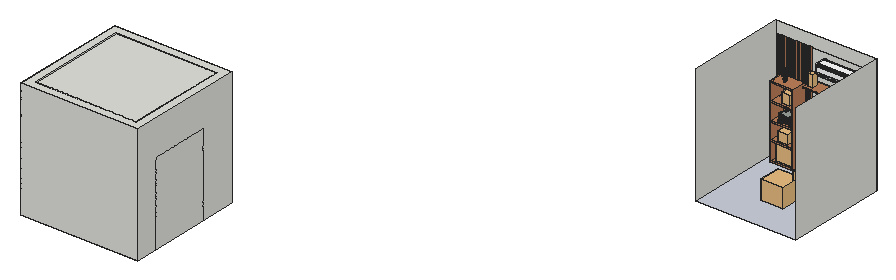
# SketchUp Ruby script. Lengths in inches.
U = 1.inch
M = Sketchup.active_model
def pt(a) = Geom::Point3d.new(a.map { |v| v * U })
def face(e, loops, mat)
  f = e.add_face(loops[0].map { |a| pt(a) })
  loops[1..].each { |l| e.add_face(l.map { |a| pt(a) }).erase! }
  f.material = f.back_material = mat if mat
  f
end
# faces: each face lists its corners as indices into pts; further lists are holes
def faces(e, pts, list, mat = nil) = list.each { |f| face(e, (f[0].is_a?(Array) ? f : [f]).map { |l| l.map { |i| pts[i] } }, mat) }
# xy, xz, yz: faces in a plane at the given z, y or x. An outline is a flat list of corners, or four numbers for a rectangle; further outlines are holes
def ring(l) = l.size == 4 ? [[l[0], l[1]], [l[2], l[1]], [l[2], l[3]], [l[0], l[3]]] : l.each_slice(2).to_a
def flat(e, list, mat, &to3) = list.each { |f| face(e, (f[0].is_a?(Array) ? f : [f]).map { |l| ring(l).map { |u, v| to3.(u, v) } }, mat) }
def xy(e, z, list, mat = nil) = flat(e, list, mat) { |x, y| [x, y, z] }
def xz(e, y, list, mat = nil) = flat(e, list, mat) { |x, z| [x, y, z] }
def yz(e, x, list, mat = nil) = flat(e, list, mat) { |y, z| [x, y, z] }
def lines(e, pts, list) = list.each { |a, b| e.add_line(pt(pts[a]), pt(pts[b])) }
# prism: a flat outline (further loops are holes) pulled along v
def prism(e, loops, v, mat = nil)
  f = face(e, loops, mat); d = Geom::Vector3d.new(v.map { |x| x * U })
  f.pushpull(f.normal.samedirection?(d) ? d.length : -d.length)
end
def box(e, o, s, mat = nil) = prism(e, [[o, [o[0] + s[0], o[1], o[2]], [o[0] + s[0], o[1] + s[1], o[2]], [o[0], o[1] + s[1], o[2]]]], [0, 0, s[2]], mat)
def at(x, y, z, deg = 0) = Geom::Transformation.translation(pt([x, y, z])) * Geom::Transformation.rotation(ORIGIN, Z_AXIS, deg.degrees)
def axes(o, x, y, z) = Geom::Transformation.new([*x, 0, *y, 0, *z, 0, *pt(o).to_a, 1])
def part(name) = M.definitions.add(name)
# library, detail: a bought-in or finely detailed component or shape, given as its bounding box
def library(name, o, s) = part(name).tap { |d| box(d.entities, o, s) }
def detail(e, o, s) = box(e.add_group.entities, o, s)
def put(e, d, t, mat = nil) = e.add_instance(d, t).tap { |i| i.material = mat if mat }
def group(e, t, mat = nil) = e.add_group.tap { |g| g.transformation = t; g.material = mat if mat }.entities
root = M.entities
M.materials.add("Book").color = [224, 222, 217]
M.materials.add("Color_000").color = [255, 255, 255]
M.materials.add("Gold_14k").color = [241, 247, 187]
M.materials.add("PDM_Books_04_Charcoal").color = [35, 35, 35]
M.materials.add("PDM_Books_04_Color_000").color = [255, 255, 255]
M.materials.add("PDM_Books_04_Color_D05").color = [255, 242, 204]
M.materials.add("PDM_Books_04_Material27").color = [78, 78, 71]
M.materials.add("PDM_Books_04_Material30").color = [128, 128, 127]
M.materials.add("PDM_Books_04_Material36").color = [212, 187, 166]
M.materials.add("PDM_Books_04_Material37").color = [155, 160, 155]
M.materials.add("PDM_Books_04_Material8").color = [90, 92, 88]
M.materials.add("[Color A05]").color = [234, 230, 226]
M.materials.add("[Color C02]").color = [238, 236, 225]
M.materials.add("[Color M06]").color = [86, 86, 86]
M.materials.add("[Color M09]").color = [0, 0, 0]
M.materials.add("[Color_A04]").color = [219, 164, 177]
M.materials.add("[Marble Carrara Floor Tile]").color = [204, 208, 219]
M.materials.add("[Wood Floor Dark]").color = [153, 94, 42]
M.materials.add("[Wood Veneer 02]").color = [190, 128, 91]
M.materials.add("bottom").color = [86, 95, 57]
c1 = library("download?mid=50c7180b9fccec56d493bfe20f94b6ab&ctyp=sp&cv=p8.",[149.43,43.83,17.86],[74.75,0.57,42.04])
c2 = library("Round+Table",[-6.7,-7.16,0],[19.69,19.69,24.5])
c3 = library("flowerpot",[-48.68,-51.05,0],[97.36,102.1,118.11])
c4 = part("Books_04_component_01")
xy(c4.entities,0,[[0.04,0,0,0.04,0,7.875,0.12,7.875,0.12,0.24,1.25,0.24,1.25,7.875,1.36,7.875,1.36,0.04,1.3125,0]],"PDM_Books_04_Color_000")
xy(c4.entities,0.11,[[0.12,0.24,0.12,7.76,0.21,7.74,0.3,7.73,0.4,7.73,0.49,7.72,0.87,7.72,0.96,7.73,1.06,7.73,1.15,7.74,1.25,7.76,1.25,0.24]],"PDM_Books_04_Color_D05")
xy(c4.entities,8.99,[[0.12,0.12,1.25,0.12,1.25,7.76,1.15,7.74,1.06,7.73,0.96,7.73,0.87,7.72,0.49,7.72,0.4,7.73,0.3,7.73,0.21,7.74,0.12,7.76]],"PDM_Books_04_Color_D05")
xy(c4.entities,9.1,[[0.04,0,1.3125,0,1.36,0.04,1.36,7.875,1.25,7.875,1.25,0.12,0.12,0.12,0.12,7.875,0,7.875,0,0.04]],"PDM_Books_04_Color_000")
xz(c4.entities,0,[[0.04,0,1.3125,9.1]],"PDM_Books_04_Material36")
xz(c4.entities,0.12,[[0.12,8.99,1.25,9.1]],"PDM_Books_04_Color_000")
xz(c4.entities,0.24,[[0.12,0,1.25,0.11]],"PDM_Books_04_Color_000")
xz(c4.entities,7.72,[[0.49,0.11,0.59,8.99],[0.59,0.11,0.68,8.99],[0.68,0.11,0.78,8.99],[0.78,0.11,0.87,8.99]],"PDM_Books_04_Color_D05")
xz(c4.entities,7.73,[[0.3,0.11,0.4,8.99],[0.96,0.11,1.06,8.99]],"PDM_Books_04_Color_D05")
xz(c4.entities,7.875,[[0,0,0.12,9.1],[1.25,0,1.36,9.1]],"PDM_Books_04_Color_000")
yz(c4.entities,0,[[0.04,0,7.875,9.1]],"PDM_Books_04_Material36")
yz(c4.entities,0.12,[[0.24,0,7.875,0,7.875,9.1,0.12,9.1,0.12,8.99,7.76,8.99,7.76,0.11,0.24,0.11]],"PDM_Books_04_Color_000")
yz(c4.entities,1.25,[[0.24,0,0.24,0.11,7.76,0.11,7.76,8.99,0.12,8.99,0.12,9.1,7.875,9.1,7.875,0]],"PDM_Books_04_Color_000")
yz(c4.entities,1.36,[[0.04,0,7.875,9.1]],"PDM_Books_04_Material36")
p = [[0.04,0,0],[0.04,0,9.1],[0,0.04,9.1],[0,0.04,0],[1.3125,0,9.1],[1.3125,0,0],
  [1.36,0.04,0],[1.36,0.04,9.1],[0.21,7.74,0.11],[0.12,7.76,0.11],[0.12,7.76,8.99],[0.21,7.74,8.99],
  [0.3,7.73,0.11],[0.3,7.73,8.99],[0.49,7.72,0.11],[0.4,7.73,0.11],[0.4,7.73,8.99],[0.49,7.72,8.99],
  [0.96,7.73,0.11],[0.87,7.72,0.11],[0.87,7.72,8.99],[0.96,7.73,8.99],[1.15,7.74,0.11],[1.06,7.73,0.11],
  [1.06,7.73,8.99],[1.15,7.74,8.99],[1.25,7.76,0.11],[1.25,7.76,8.99]]
faces(c4.entities,p,[[0,1,2,3],[4,5,6,7]],"PDM_Books_04_Material36")
faces(c4.entities,p,[[8,9,10,11],[12,8,11,13],[14,15,16,17],[18,19,20,21],[22,23,24,25],[26,22,25,27]],"PDM_Books_04_Color_D05")
c5 = part("Books_04_component_05")
xy(c5.entities,0,[[0.04,0,0,0.04,0,8.31,0.12,8.31,0.12,0.24,0.83,0.18,0.83,8.31,0.94,8.31,0.94,0.04,0.9,0]],"PDM_Books_04_Color_000")
xy(c5.entities,0.11,[[0.83,0.18,0.12,0.24,0.12,8.1875,0.17,8.18,0.23,8.18,0.29,8.17,0.35,8.17,0.41,8.16,0.53,8.16,0.59,8.17,0.65,8.17,0.71,8.18,0.77,8.18,0.83,8.1875]],"PDM_Books_04_Color_D05")
xy(c5.entities,9.65,[[0.12,0.24,0.83,0.24,0.83,8.1875,0.77,8.18,0.71,8.18,0.65,8.17,0.59,8.17,0.53,8.16,0.41,8.16,0.35,8.17,0.29,8.17,0.23,8.18,0.17,8.18,0.12,8.1875]],"PDM_Books_04_Color_D05")
xy(c5.entities,9.76,[[0.04,0,0.9,0,0.94,0.04,0.94,8.31,0.83,8.31,0.83,0.24,0.12,0.24,0.12,8.31,0,8.31,0,0.04]],"PDM_Books_04_Color_000")
xz(c5.entities,0,[[0.04,0,0.9,9.76]],"PDM_Books_04_Material37")
xz(c5.entities,0.24,[[0.12,9.65,0.83,9.76]],"PDM_Books_04_Color_000")
xz(c5.entities,8.16,[[0.41,0.11,0.47,9.65],[0.47,0.11,0.53,9.65]],"PDM_Books_04_Color_D05")
xz(c5.entities,8.17,[[0.29,0.11,0.35,9.65],[0.59,0.11,0.65,9.65]],"PDM_Books_04_Color_D05")
xz(c5.entities,8.18,[[0.17,0.11,0.23,9.65],[0.71,0.11,0.77,9.65]],"PDM_Books_04_Color_D05")
xz(c5.entities,8.31,[[0,0,0.12,9.76],[0.83,0,0.94,9.76]],"PDM_Books_04_Color_000")
yz(c5.entities,0,[[0.04,0,8.31,9.76]],"PDM_Books_04_Material37")
yz(c5.entities,0.12,[[0.24,0,8.31,0,8.31,9.76,0.24,9.76,0.24,9.65,8.1875,9.65,8.1875,0.11,0.24,0.11]],"PDM_Books_04_Color_000")
yz(c5.entities,0.83,[[0.18,0,0.18,0.11,8.1875,0.11,8.1875,9.65,0.24,9.65,0.24,9.76,8.31,9.76,8.31,0]],"PDM_Books_04_Color_000")
yz(c5.entities,0.94,[[0.04,0,8.31,9.76]],"PDM_Books_04_Material37")
p = [[0,0.04,9.76],[0,0.04,0],[0.04,0,0],[0.04,0,9.76],[0.94,0.04,0],[0.94,0.04,9.76],
  [0.9,0,9.76],[0.9,0,0],[0.83,0.18,0.11],[0.83,0.18,0],[0.12,0.24,0],[0.12,0.24,0.11],
  [0.12,8.1875,0.11],[0.12,8.1875,9.65],[0.17,8.18,9.65],[0.17,8.18,0.11],[0.29,8.17,0.11],[0.23,8.18,0.11],
  [0.23,8.18,9.65],[0.29,8.17,9.65],[0.41,8.16,0.11],[0.35,8.17,0.11],[0.35,8.17,9.65],[0.41,8.16,9.65],
  [0.59,8.17,0.11],[0.53,8.16,0.11],[0.53,8.16,9.65],[0.59,8.17,9.65],[0.71,8.18,0.11],[0.65,8.17,0.11],
  [0.65,8.17,9.65],[0.71,8.18,9.65],[0.83,8.1875,0.11],[0.77,8.18,0.11],[0.77,8.18,9.65],[0.83,8.1875,9.65]]
faces(c5.entities,p,[[0,1,2,3],[4,5,6,7]],"PDM_Books_04_Material37")
faces(c5.entities,p,[[8,9,10,11]],"PDM_Books_04_Color_000")
faces(c5.entities,p,[[12,13,14,15],[16,17,18,19],[20,21,22,23],[24,25,26,27],[28,29,30,31],[32,33,34,35]],"PDM_Books_04_Color_D05")
c6 = part("Books_04_component_02")
xy(c6.entities,0,[[0.04,0,0,0.04,0,7.67,0.12,7.67,0.12,0.12,1.11,0.12,1.11,7.67,1.22,7.67,1.22,0.04,1.18,0]],"PDM_Books_04_Color_000")
xy(c6.entities,0.08,[[0.12,0.12,1.11,7.59]],"PDM_Books_04_Color_D05")
xy(c6.entities,10.875,[[0.12,0.12,1.11,7.59]],"PDM_Books_04_Color_D05")
xy(c6.entities,10.99,[[0.04,0,1.18,0,1.22,0.04,1.22,7.67,1.11,7.67,1.11,0.12,0.12,0.12,0.12,7.67,0,7.67,0,0.04]],"PDM_Books_04_Color_000")
xz(c6.entities,0,[[0.04,0,1.18,10.99]],"PDM_Books_04_Material8")
xz(c6.entities,0.12,[[0.12,0,1.11,0.08],[0.12,0.08,1.11,10.875]])
xz(c6.entities,0.12,[[0.12,10.875,1.11,10.99]],"PDM_Books_04_Color_000")
xz(c6.entities,7.59,[[0.12,0.08,1.11,10.875]],"PDM_Books_04_Color_D05")
xz(c6.entities,7.67,[[1.11,0,1.22,10.99]],"PDM_Books_04_Color_000")
xz(c6.entities,7.67,[[0,0,0.12,10.99]],"PDM_Books_04_Material8")
yz(c6.entities,0,[[0.04,0,7.67,10.99]],"PDM_Books_04_Material8")
yz(c6.entities,0.12,[[0.12,0,7.67,0,7.67,10.99,0.12,10.99,0.12,10.875,7.59,10.875,7.59,0.08,0.12,0.08]])
yz(c6.entities,0.12,[[0.12,0.08,7.59,10.875]],"PDM_Books_04_Material8")
yz(c6.entities,1.11,[[0.12,0,0.12,0.08,7.59,0.08,7.59,10.875,0.12,10.875,0.12,10.99,7.67,10.99,7.67,0],[0.12,0.08,7.59,10.875]])
yz(c6.entities,1.22,[[0.04,0,7.67,10.99]],"PDM_Books_04_Material8")
p = [[0,0.04,10.99],[0,0.04,0],[0.04,0,0],[0.04,0,10.99],[1.22,0.04,0],[1.22,0.04,10.99],
  [1.18,0,10.99],[1.18,0,0]]
faces(c6.entities,p,[[0,1,2,3],[4,5,6,7]],"PDM_Books_04_Material8")
c7 = part("Books_04_component_03")
xy(c7.entities,0,[[0.04,0,0,0.04,0,7.67,0.12,7.67,0.12,0.12,1.11,0.12,1.11,7.67,1.22,7.67,1.22,0.04,1.18,0]],"PDM_Books_04_Color_000")
xy(c7.entities,0.08,[[0.12,0.12,1.11,7.59]],"PDM_Books_04_Color_D05")
xy(c7.entities,9.89,[[0.12,0.12,1.11,7.59]],"PDM_Books_04_Color_D05")
xy(c7.entities,10,[[0.04,0,1.18,0,1.22,0.04,1.22,7.67,1.11,7.67,1.11,0.12,0.12,0.12,0.12,7.67,0,7.67,0,0.04]],"PDM_Books_04_Color_000")
xz(c7.entities,0,[[0.04,7.99,1.18,10]],"PDM_Books_04_Color_000")
xz(c7.entities,0,[[0.04,0,1.18,7.99]],"PDM_Books_04_Material30")
xz(c7.entities,0.12,[[0.12,0,1.11,0.08],[0.12,0.08,1.11,9.89]])
xz(c7.entities,0.12,[[0.12,9.89,1.11,10]],"PDM_Books_04_Color_000")
xz(c7.entities,7.59,[[0.12,0.08,1.11,9.89]],"PDM_Books_04_Color_D05")
xz(c7.entities,7.67,[[1.11,0,1.22,10]],"PDM_Books_04_Color_000")
xz(c7.entities,7.67,[[0,0,0.12,10]],"PDM_Books_04_Material8")
yz(c7.entities,0,[[0.04,0,7.67,10]],"PDM_Books_04_Material30")
yz(c7.entities,0.12,[[0.12,0,7.67,0,7.67,10,0.12,10,0.12,9.89,7.59,9.89,7.59,0.08,0.12,0.08]])
yz(c7.entities,0.12,[[0.12,0.08,7.59,9.89]],"PDM_Books_04_Material8")
yz(c7.entities,1.11,[[0.12,0,0.12,0.08,7.59,0.08,7.59,9.89,0.12,9.89,0.12,10,7.67,10,7.67,0],[0.12,0.08,7.59,9.89]])
yz(c7.entities,1.22,[[0.04,0,7.67,10]],"PDM_Books_04_Material30")
p = [[0.04,0,0],[0.04,0,7.99],[0,0.04,7.99],[0,0.04,0],[1.18,0,7.99],[1.18,0,0],
  [1.22,0.04,0],[1.22,0.04,7.99],[0.04,0,10],[0,0.04,10],[1.18,0,10],[1.22,0.04,10]]
faces(c7.entities,p,[[0,1,2,3],[4,5,6,7]],"PDM_Books_04_Material30")
faces(c7.entities,p,[[1,8,9,2],[10,4,7,11]],"PDM_Books_04_Color_000")
c8 = part("Books_04_component_04")
xy(c8.entities,0,[[0.04,0,0,0.04,0,8.1,0.12,8.1,0.12,0.12,1.11,0.12,1.11,8.1,1.22,8.1,1.22,0.04,1.18,0]],"PDM_Books_04_Color_000")
xy(c8.entities,0.08,[[0.12,0.12,1.11,8.02]],"PDM_Books_04_Color_D05")
xy(c8.entities,11.98,[[0.12,0.12,1.11,8.02]],"PDM_Books_04_Color_D05")
xy(c8.entities,12.09,[[0.04,0,1.18,0,1.22,0.04,1.22,8.1,1.11,8.1,1.11,0.12,0.12,0.12,0.12,8.1,0,8.1,0,0.04]],"PDM_Books_04_Color_000")
xz(c8.entities,0,[[0.04,7.96,1.18,12.09]],"PDM_Books_04_Charcoal")
xz(c8.entities,0,[[0.04,0,1.18,7.96]],"PDM_Books_04_Material27")
xz(c8.entities,0.12,[[0.12,0,1.11,0.08],[0.12,0.08,1.11,11.98]])
xz(c8.entities,0.12,[[0.12,11.98,1.11,12.09]],"PDM_Books_04_Color_000")
xz(c8.entities,8.02,[[0.12,0.08,1.11,11.98]],"PDM_Books_04_Color_D05")
xz(c8.entities,8.1,[[1.11,0,1.22,12.09]],"PDM_Books_04_Color_000")
xz(c8.entities,8.1,[[0,0,0.12,12.09]],"PDM_Books_04_Material8")
yz(c8.entities,0,[[0.04,0,8.1,12.09]],"PDM_Books_04_Material27")
yz(c8.entities,0.12,[[0.12,0,8.1,0,8.1,12.09,0.12,12.09,0.12,11.98,8.02,11.98,8.02,0.08,0.12,0.08]])
yz(c8.entities,0.12,[[0.12,0.08,8.02,11.98]],"PDM_Books_04_Material8")
yz(c8.entities,1.11,[[0.12,0,0.12,0.08,8.02,0.08,8.02,11.98,0.12,11.98,0.12,12.09,8.1,12.09,8.1,0],[0.12,0.08,8.02,11.98]])
yz(c8.entities,1.22,[[0.04,0,8.1,12.09]],"PDM_Books_04_Material27")
p = [[0,0.04,7.96],[0,0.04,0],[0.04,0,0],[0.04,0,7.96],[1.18,0,7.96],[1.18,0,0],
  [1.22,0.04,0],[1.22,0.04,7.96],[0,0.04,12.09],[0.04,0,12.09],[1.18,0,12.09],[1.22,0.04,12.09]]
faces(c8.entities,p,[[0,1,2,3],[4,5,6,7]],"PDM_Books_04_Material27")
faces(c8.entities,p,[[8,0,3,9],[10,4,7,11]],"PDM_Books_04_Charcoal")
c9 = part("Book")
put(c9.entities,c4,axes([4.875,-4.73,3.67],[0,0,1],[0.10106,0.99488,0],[-0.99488,0.10106,0]))
put(c9.entities,c5,axes([4.5,-4.91,5.03],[0,0,1],[0.17365,0.98481,0],[-0.98481,0.17365,0]))
put(c9.entities,c6,axes([4.85,-4.7,1.22],[0,0,1],[0.108,0.99415,0],[-0.99415,0.108,0]))
put(c9.entities,c7,axes([5.47,-3.69,2.45],[0,0,1],[-0.04711,0.99889,0],[-0.99889,-0.04711,0]))
put(c9.entities,c8,axes([6.6,-3.07,0],[0,0,1],[-0.15643,0.98769,0],[-0.98769,-0.15643,0]))
c10 = library("Vase with Flower",[-2.59,-2.59,0],[5.18,5.18,11.38])
c11 = part("stem")
p = [[8.92,1.38,83.34],[12.34,1.73,96.125],[8.32,0.48,83.4375],[8.19,2.35,83.4375],[11.85,2.6,96.21],[6.99,0.55,83.63],
  [10.86,0.86,96.39],[11.85,0.86,96.21],[6.86,2.43,83.63],[10.86,2.6,96.39],[6.26,1.53,83.73],[10.36,1.73,96.48],
  [16.61,1.73,120.56],[16.3,1.18,120.63],[16.3,2.28,120.63],[15.69,1.18,120.77],[15.69,2.28,120.77],[15.375,1.73,120.84],
  [21.36,1.47,144.07],[21.11,1.47,144.13],[21.49,1.6875,144.05],[21.36,1.91,144.07],[21.11,1.91,144.13],[20.99,1.6875,144.16]]
faces(c11.entities,p,[[0,1,2],[3,4,0],[1,0,4],[5,2,6],[7,2,1],[7,6,2],[8,9,3],[4,3,9],
  [5,6,10],[8,10,9],[11,10,6],[11,9,10],[7,1,12,13],[1,4,14,12],[7,13,15,6],[4,9,16,14],
  [6,15,17,11],[17,16,9,11],[18,19,15,13],[12,20,18,13],[20,12,14,21],[21,14,16,22],[19,23,17,15],[16,17,23,22]],"bottom")
faces(c11.entities,p,[[18,20,21,22,23,19]])
c12 = part("leaf")
xy(c12.entities,0,[[1.27,0.625,0,1.89,0,3.7,1.27,5.43,3.34,6.6875,3.34,1.02]],"bottom")
p = [[3.34,6.6875,0],[5.69,5.05,-0.75],[6.53,3.7,-1.02],[6.53,1.64,-1.02],[4.9375,0.625,-0.51],[3.34,1.02,0],
  [3.34,0.4375,0],[3.34,0,0]]
faces(c12.entities,p,[[0,1,2,3,4,5]],"bottom")
lines(c12.entities,p,[[5,6],[6,7]])
c13 = part("petal\#1")
p = [[0.59,-0.98,-0.45],[0.74,-1.1,-0.29],[0.41,-0.67,-0.14],[0.42,-0.77,-0.38],[1.2,-1.19,-0.06],[0.54,-0.34,0.24],
  [1.12,0.01,0.5],[1.78,-0.84,0.21],[1.45,-0.41,0.36],[0,0.42,0],[0.09,0.28,0.2],[0.09,0.84,0.2],
  [0,0.7,0],[1.87,-0.35,0.24],[2.18,-0.15,0.17],[2.39,0.2,0.15],[2.22,0.41,0.23],[1.85,0.28,0.32],
  [1.6,0,0.36],[0.45,0,0.45],[0.45,1.12,0.45],[1.87,0.28,0.35],[1.87,0.84,0.35],[2.23,0.7,0.23],
  [1.51,0.33,0.48],[1.16,0.56,0.6],[1.16,0,0.6],[1.51,0.79,0.48],[1.16,1.12,0.6]]
faces(c13.entities,p,[[0,1,2,3],[1,4,5,2],[6,5,4,7,8],[9,10,11,12],[13,8,7,14],[14,15,16,17,18,8,13],[10,19,20,11],[21,16,22],
  [23,22,16],[6,8,18,17],[24,25,26,21],[22,27,25,24,21],[28,25,27,22],[28,20,19,26,25]],"[Color_A04]")
c14 = part("flower")
put(c14.entities,c13,axes([2.1,0,0.625],[-0.03304,0.72958,0.14199],[-0.77918,0,-0.18132],[-0.17781,-0.15676,0.76408]))
put(c14.entities,c13,axes([3.38,2.1,1.25],[-0.77918,0,-0.18132],[0,-0.8,0],[-0.18132,0,0.77918]))
put(c14.entities,c13,axes([0.01,1.2,0],[0.7057,0,0.37681],[0,0.8,0],[-0.37681,0,0.7057]))
put(c14.entities,c13,axes([1.16,3.49,0.73],[0,-0.8,0],[0.77918,0,0.18132],[-0.18132,0,0.77918]))
c15 = part("Plant_flower")
p = [[4.13,-5.21,48.5625],[2.97,-5.27,48.18],[2.1,-5.33,47.33],[1.6875,-5.39,46.18],[2.87,-8.33,51.63],[2.46,-7.41,51.49],
  [2,-6.68,50.88],[1.58,-6.29,49.94]]
lines(c15.entities,p,[[0,1],[1,2],[2,3],[4,5],[6,7],[5,6]])
put(c15.entities,c11,axes([-0.85,0.55,-1.29],[0.10275,-0.38349,0],[0.38349,0.10275,0],[0,0,0.39701]))
put(c15.entities,c12,axes([3.82,-6.52,48.84],[0.09945,0.40738,-0.08753],[0.52591,-0.18667,-0.27125],[-0.22953,-0.03449,-0.42129]))
put(c15.entities,c14,axes([6.9,-4.04,53.68],[-2.40969,0.82543,0.59906],[-0.96837,-2.33406,-0.67913],[0.32013,-0.84712,2.45494]))
put(c15.entities,c12,axes([1.64,-8.47,52.18],[0.38389,0.04123,-0.17257],[-0.11872,-0.44244,-0.27916],[-0.18424,0.2028,-0.32786]))
c16 = part("stem2")
p = [[11.85,0.86,96.21],[12.34,1.73,96.125],[16.61,1.73,120.56],[16.3,1.18,120.63],[11.85,2.6,96.21],[16.3,2.28,120.63],
  [15.69,1.18,120.77],[10.86,0.86,96.39],[10.86,2.6,96.39],[15.69,2.28,120.77],[15.375,1.73,120.84],[10.36,1.73,96.48],
  [21.36,1.47,144.07],[21.11,1.47,144.13],[21.49,1.6875,144.05],[21.36,1.91,144.07],[21.11,1.91,144.13],[20.99,1.6875,144.16]]
faces(c16.entities,p,[[0,1,2,3],[1,4,5,2],[0,3,6,7],[4,8,9,5],[7,6,10,11],[10,9,8,11],[12,13,6,3],[2,14,12,3],
  [14,2,5,15],[15,5,9,16],[13,17,10,6],[9,10,17,16]],"bottom")
faces(c16.entities,p,[[12,14,15,16,17,13]])
c17 = part("Plant_flower2")
p = [[2.87,-8.33,51.63],[2.46,-7.41,51.49],[2,-6.68,50.88],[1.58,-6.29,49.94]]
lines(c17.entities,p,[[0,1],[2,3],[1,2]])
put(c17.entities,c16,axes([-0.85,0.55,-1.29],[0.10275,-0.38349,0],[0.38349,0.10275,0],[0,0,0.39701]))
put(c17.entities,c14,axes([6.9,-4.04,53.68],[-2.40969,0.82543,0.59906],[-0.96837,-2.33406,-0.67913],[0.32013,-0.84712,2.45494]))
put(c17.entities,c12,axes([1.64,-8.47,52.18],[0.38389,0.04123,-0.17257],[-0.11872,-0.44244,-0.27916],[-0.18424,0.2028,-0.32786]))
c18 = part("Vase_Quarter\#3")
xy(c18.entities,0,[[0,0,0,0.8,0.21,0.8,0.59,0.59,0.8,0.21,0.8,0]])
xz(c18.entities,0.78,[[0,9.66,0.21,10.84]])
yz(c18.entities,0.78,[[0,9.66,0.21,10.84]])
p = [[0.8,0,0],[0.8,0.21,0],[1.35,0.42,2.81],[1.35,0,2.81],[0.59,0.59,0],[1.01,1.01,2.81],
  [0.21,0.8,0],[0.42,1.35,2.81],[0,0.8,0],[0,1.35,2.81],[1.51,0.46,4.94],[1.51,0,4.94],
  [1.125,1.125,4.94],[0.46,1.51,4.94],[0,1.51,4.94],[1.43,0.43,6.19],[1.43,0,6.19],[1.07,1.07,6.19],
  [0.43,1.43,6.19],[0,1.43,6.19],[1,0.27,8.5],[1,0,8.5],[0.73,0.73,8.5],[0.27,1,8.5],
  [0,1,8.5],[0.78,0.21,9.66],[0.78,0,9.66],[0.57,0.57,9.66],[0.21,0.78,9.66],[0,0.78,9.66],
  [0.57,0.57,10.84],[0.78,0.21,10.84],[0.21,0.78,10.84],[1,0.27,12],[1,0,12],[0.78,0,10.84],
  [0.73,0.73,12],[0.27,1,12],[0,0.78,10.84],[0,1,12]]
faces(c18.entities,p,[[0,1,2,3],[4,5,2,1],[5,4,6,7],[7,6,8,9],[2,10,11,3],[5,12,10,2],[12,5,7,13],[13,7,9,14],
  [10,15,16,11],[12,17,15,10],[12,13,18,17],[13,14,19,18],[15,20,21,16],[17,22,20,15],[17,18,23,22],[18,19,24,23],
  [25,26,21,20],[22,27,25,20],[23,28,27,22],[23,24,29,28],[27,30,31,25],[28,32,30,27],[33,34,35,31],[30,36,33,31],
  [32,37,36,30],[32,38,39,37]])
c19 = part("vase_thin\#1")
put(c19.entities,c18,at(0,0,0))
put(c19.entities,c18,at(0,0,0,90))
put(c19.entities,c18,at(0,0,0,180))
put(c19.entities,c18,at(0,0,0,-90))
c20 = part("Vase with flowers")
put(c20.entities,c15,axes([3.625,2.02,-8.35],[-0.06695,-0.33202,0.02963],[0.33329,-0.0672,0],[0.00586,0.02905,0.33871]))
put(c20.entities,c15,axes([1.32,2.29,-9.75],[-0.088,0.32841,0],[-0.32841,-0.088,0],[0,0,0.34]))
put(c20.entities,c17,axes([3.73,4.01,-12],[0.14851,-0.30585,0],[0.30585,0.14851,0],[0,0,0.34]))
put(c20.entities,c19,axes([2.72,2.71,0],[1,0,0],[0,1,0],[0,0,0.44]))
put(c20.entities,c15,axes([2.75,3.98,-10.5],[0.33881,-0.02845,0],[0.02845,0.33881,0],[0,0,0.34]))
c21 = library("007",[-7.44,-2.67,-4.4375],[12.18,12.03,12.77])
c22 = library("skpE36B",[-3.84,-2.73,0],[7.68,5.46,1.59])
c23 = library("skpA613",[-33.11,-37.89,-86.79],[66.22,75.78,173.58])
c24 = library("Row of books",[-2.76,0,0],[10.13,7.78,9.38])
c25 = part("Open-Book2")
g1 = group(c25.entities,at(-83.63,0.99,-0.02))
g2 = group(g1,at(0,0,0))
xy(g2,0.028,[[0,0,2.913,10.029],[12.526,0,16.143,10.029]],"[Color M06]")
xy(g2,0.271,[[0.25,0,2.855,10.029]],"[Color A05]")
xy(g2,0.528,[[12.444,0,15.85,10.029]],"[Color C02]")
xz(g2,0,[[8.098,0,8.236,0.143,8.389,0.271,8.554,0.383,8.729,0.477,8.914,0.553,9.105,0.609,9.301,0.645,9.5,0.66,9.639,0.657,9.699,0.655,9.896,0.63,10.09,0.584,10.278,0.519,11,0.313,11.754,0.123,12.526,0.028,16.143,0.028,15.85,0.528,12.444,0.528,11.844,0.602,11.126,0.783,10.855,0.929,10.57,1.046,10.275,1.133,9.972,1.187,9.665,1.209,9.357,1.199,9.0625,1.158,9.052,1.156,8.753,1.082,8.464,0.976,8.1875,0.84,7.927,0.676,7.685,0.485,7.594,0.824,7.484,1.058,7.3,1.302,7.07,1.503,6.804,1.653,6.636,1.672,6.467,1.678,6.298,1.672,6.13,1.652,5.963,1.62,5.8,1.574,5.641,1.517,5.487,1.447,5.338,1.365,5.197,1.272,5.063,1.169,4.937,1.055,4.775,0.963,4.611,0.875,4.451,0.795,4.444,0.792,4.284,0.706,3.933,0.574,3.93,0.573,3.928,0.572,3.592,0.445,3.414,0.403,3.399,0.398,3.219,0.351,3.038,0.308,2.855,0.271,0.25,0.271,0,0.028,2.913,0.028,3.661,0.204,3.665,0.205,3.669,0.207,4.383,0.477,4.388,0.478,4.392,0.481,5.066,0.841,5.072,0.845,5.698,1.292,5.784,1.355,5.876,1.409,5.973,1.454,6.074,1.488,6.178,1.512,6.243,1.521,6.253,1.525,6.262,1.523,6.284,1.526,6.391,1.528,6.497,1.52,6.602,1.501,6.705,1.471,6.804,1.432,6.819,1.423,6.867,1.398,6.898,1.382,6.987,1.323,7.07,1.255,7.145,1.179,7.212,1.096,7.245,1.045,7.27,1.007,7.299,0.951,7.319,0.912,7.358,0.8125,7.387,0.71,7.405,0.605,7.413,0.498,7.413,0.497,7.409,0.391,7.395,0.286,7.37,0.182]],"Book")
xz(g2,10.029,[[8.098,0,7.37,0.182,7.395,0.286,7.409,0.391,7.413,0.497,7.413,0.498,7.405,0.605,7.387,0.71,7.358,0.8125,7.319,0.912,7.299,0.951,7.27,1.007,7.245,1.045,7.212,1.096,7.145,1.179,7.07,1.255,6.987,1.323,6.898,1.382,6.867,1.398,6.819,1.423,6.804,1.432,6.705,1.471,6.602,1.501,6.497,1.52,6.391,1.528,6.284,1.526,6.262,1.523,6.253,1.525,6.243,1.521,6.178,1.512,6.074,1.488,5.973,1.454,5.876,1.409,5.784,1.355,5.698,1.292,5.072,0.845,5.066,0.841,4.392,0.481,4.388,0.478,4.383,0.477,3.669,0.207,3.665,0.205,3.661,0.204,2.913,0.028,0,0.028,0.25,0.271,2.855,0.271,3.038,0.308,3.219,0.351,3.399,0.398,3.414,0.403,3.592,0.445,3.928,0.572,3.93,0.573,3.933,0.574,4.284,0.706,4.444,0.792,4.451,0.795,4.611,0.875,4.775,0.963,4.937,1.055,5.063,1.169,5.197,1.272,5.338,1.365,5.487,1.447,5.641,1.517,5.8,1.574,5.963,1.62,6.13,1.652,6.298,1.672,6.467,1.678,6.636,1.672,6.804,1.653,7.07,1.503,7.3,1.302,7.484,1.058,7.594,0.824,7.685,0.485,7.927,0.676,8.1875,0.84,8.464,0.976,8.753,1.082,9.052,1.156,9.0625,1.158,9.357,1.199,9.665,1.209,9.972,1.187,10.275,1.133,10.57,1.046,10.855,0.929,11.126,0.783,11.844,0.602,12.444,0.528,15.85,0.528,16.143,0.028,12.526,0.028,11.754,0.123,11,0.313,10.278,0.519,10.09,0.584,9.896,0.63,9.699,0.655,9.639,0.657,9.5,0.66,9.301,0.645,9.105,0.609,8.914,0.553,8.729,0.477,8.554,0.383,8.389,0.271,8.236,0.143]],"Book")
yz(g2,7.413,[[0,0.497,10.029,0.498]],"[Color M06]")
p = [[0,0,0.028],[0.25,0,0.271],[0.25,10.029,0.271],[0,10.029,0.028],[3.661,0,0.204],[2.913,0,0.028],
  [2.913,10.029,0.028],[3.661,10.029,0.204],[8.098,0,0],[7.37,0,0.182],[7.37,10.029,0.182],[8.098,10.029,0],
  [8.236,0,0.143],[8.236,10.029,0.143],[12.526,0,0.028],[11.754,0,0.123],[11.754,10.029,0.123],[12.526,10.029,0.028],
  [15.85,0,0.528],[16.143,0,0.028],[16.143,10.029,0.028],[15.85,10.029,0.528],[8.389,0,0.271],[8.389,10.029,0.271],
  [11,0,0.313],[11,10.029,0.313],[3.665,0,0.205],[3.665,10.029,0.205],[3.669,0,0.207],[3.669,10.029,0.207],
  [4.383,0,0.477],[4.383,10.029,0.477],[7.395,0,0.286],[7.395,10.029,0.286],[2.855,0,0.271],[3.038,0,0.308],
  [3.038,10.029,0.308],[2.855,10.029,0.271],[3.219,0,0.351],[3.219,10.029,0.351],[7.409,0,0.391],[7.409,10.029,0.391],
  [8.554,0,0.383],[8.554,10.029,0.383],[10.278,0,0.519],[10.278,10.029,0.519],[3.399,0,0.398],[3.399,10.029,0.398],
  [3.414,0,0.403],[3.592,0,0.445],[3.592,10.029,0.445],[3.414,10.029,0.403],[3.928,0,0.572],[3.928,10.029,0.572],
  [7.413,0,0.497],[7.413,10.029,0.497],[8.729,0,0.477],[8.729,10.029,0.477],[4.388,0,0.478],[4.388,10.029,0.478],
  [4.392,0,0.481],[4.392,10.029,0.481],[5.066,0,0.841],[5.066,10.029,0.841],[7.413,0,0.498],[7.405,0,0.605],
  [7.405,10.029,0.605],[7.413,10.029,0.498],[7.594,0,0.824],[7.685,0,0.485],[7.685,10.029,0.485],[7.594,10.029,0.824],
  [7.927,0,0.676],[7.927,10.029,0.676],[8.914,0,0.553],[8.914,10.029,0.553],[10.09,0,0.584],[10.09,10.029,0.584],
  [11.844,0,0.602],[12.444,0,0.528],[12.444,10.029,0.528],[11.844,10.029,0.602],[3.933,0,0.574],[4.284,0,0.706],
  [4.284,10.029,0.706],[3.933,10.029,0.574],[3.93,0,0.573],[3.93,10.029,0.573],[7.387,0,0.71],[7.387,10.029,0.71],
  [9.105,0,0.609],[9.105,10.029,0.609],[9.301,0,0.645],[9.301,10.029,0.645],[9.5,0,0.66],[9.5,10.029,0.66],
  [9.896,0,0.63],[9.699,0,0.655],[9.699,10.029,0.655],[9.896,10.029,0.63],[11.126,0,0.783],[11.126,10.029,0.783],
  [4.444,0,0.792],[4.444,10.029,0.792],[7.358,0,0.8125],[7.358,10.029,0.8125],[8.1875,0,0.84],[8.1875,10.029,0.84],
  [9.639,0,0.657],[9.639,10.029,0.657],[4.451,0,0.795],[4.451,10.029,0.795],[4.611,0,0.875],[4.611,10.029,0.875],
  [5.069,0,0.843],[5.069,10.029,0.843],[5.072,0,0.845],[5.072,10.029,0.845],[5.698,0,1.292],[5.698,10.029,1.292],
  [7.319,0,0.912],[7.319,10.029,0.912],[7.484,0,1.058],[7.484,10.029,1.058],[8.464,0,0.976],[8.464,10.029,0.976],
  [10.855,0,0.929],[10.855,10.029,0.929],[4.775,0,0.963],[4.775,10.029,0.963],[7.299,0,0.951],[7.299,10.029,0.951],
  [10.57,0,1.046],[10.57,10.029,1.046],[4.937,0,1.055],[4.937,10.029,1.055],[7.245,0,1.045],[7.212,0,1.096],
  [7.212,10.029,1.096],[7.245,10.029,1.045],[7.27,0,1.007],[7.27,10.029,1.007],[8.753,0,1.082],[8.753,10.029,1.082],
  [10.275,0,1.133],[10.275,10.029,1.133],[5.063,0,1.169],[5.063,10.029,1.169],[7.145,0,1.179],[7.145,10.029,1.179],
  [7.3,0,1.302],[7.3,10.029,1.302],[9.052,0,1.156],[9.052,10.029,1.156],[9.972,0,1.187],[9.972,10.029,1.187],
  [5.197,0,1.272],[5.197,10.029,1.272],[7.07,0,1.255],[7.07,10.029,1.255],[9.0625,0,1.158],[9.357,0,1.199],
  [9.357,10.029,1.199],[9.0625,10.029,1.158],[9.665,0,1.209],[9.665,10.029,1.209],[5.338,0,1.365],[5.338,10.029,1.365],
  [5.784,0,1.355],[5.784,10.029,1.355],[6.987,0,1.323],[6.898,0,1.382],[6.898,10.029,1.382],[6.987,10.029,1.323],
  [7.07,0,1.503],[7.07,10.029,1.503],[5.487,0,1.447],[5.487,10.029,1.447],[5.641,0,1.517],[5.641,10.029,1.517],
  [5.876,0,1.409],[5.876,10.029,1.409],[5.973,0,1.454],[5.973,10.029,1.454],[6.804,0,1.432],[6.705,0,1.471],
  [6.705,10.029,1.471],[6.804,10.029,1.432],[6.819,0,1.423],[6.819,10.029,1.423],[6.867,0,1.398],[6.867,10.029,1.398],
  [5.8,0,1.574],[5.8,10.029,1.574],[6.074,0,1.488],[6.074,10.029,1.488],[6.178,0,1.512],[6.178,10.029,1.512],
  [6.243,0,1.521],[6.243,10.029,1.521],[6.253,0,1.525],[6.253,10.029,1.525],[6.262,0,1.523],[6.262,10.029,1.523],
  [6.284,0,1.526],[6.284,10.029,1.526],[6.391,0,1.528],[6.391,10.029,1.528],[6.497,0,1.52],[6.497,10.029,1.52],
  [6.602,0,1.501],[6.602,10.029,1.501],[6.804,0,1.653],[6.804,10.029,1.653],[5.963,0,1.62],[5.963,10.029,1.62],
  [6.13,0,1.652],[6.13,10.029,1.652],[6.298,0,1.672],[6.298,10.029,1.672],[6.467,0,1.678],[6.467,10.029,1.678],
  [6.636,0,1.672],[6.636,10.029,1.672]]
faces(g2,p,[[0,1,2,3],[18,19,20,21]],"Book")
faces(g2,p,[[4,5,6,7],[8,9,10,11],[12,8,11,13],[14,15,16,17],[22,12,13,23],[15,24,25,16],[26,4,7,27],[28,26,27,29],
  [30,28,29,31],[9,32,33,10],[32,40,41,33],[42,22,23,43],[24,44,45,25],[40,54,55,41],[56,42,43,57],[58,30,31,59],
  [60,58,59,61],[62,60,61,63],[64,65,66,67],[74,56,57,75],[44,76,77,45],[65,88,89,66],[90,74,75,91],[92,90,91,93],
  [94,92,93,95],[96,97,98,99],[76,96,99,77],[88,104,105,89],[108,94,95,109],[97,108,109,98],[114,62,63,115],[116,114,115,117],
  [118,116,117,119],[104,120,121,105],[120,130,131,121],[136,137,138,139],[140,136,139,141],[130,140,141,131],[137,148,149,138],[148,158,159,149],
  [168,118,119,169],[170,171,172,173],[158,170,173,159],[180,168,169,181],[182,180,181,183],[184,185,186,187],[188,184,187,189],[190,188,189,191],
  [171,190,191,172],[194,182,183,195],[196,194,195,197],[198,196,197,199],[200,198,199,201],[202,200,201,203],[204,202,203,205],[206,204,205,207],
  [208,206,207,209],[210,208,209,211],[185,210,211,186]],"[Color M06]")
faces(g2,p,[[34,35,36,37],[35,38,39,36],[38,46,47,39],[48,49,50,51],[46,48,51,47],[49,52,53,50],[68,69,70,71],[82,83,84,85],
  [86,82,85,87],[52,86,87,53],[83,102,103,84],[102,110,111,103],[110,112,113,111],[122,68,71,123],[112,128,129,113],[128,134,135,129],
  [134,146,147,135],[150,122,123,151],[146,156,157,147],[156,166,167,157],[174,150,151,175],[166,176,177,167],[176,178,179,177],[178,192,193,179],
  [212,174,175,213],[192,214,215,193],[214,216,217,215],[216,218,219,217],[218,220,221,219],[220,222,223,221],[222,212,213,223]],"[Color A05]")
faces(g2,p,[[69,72,73,70],[78,79,80,81],[100,78,81,101],[72,106,107,73],[106,124,125,107],[126,100,101,127],[132,126,127,133],[124,142,143,125],
  [144,132,133,145],[142,152,153,143],[154,144,145,155],[160,161,162,163],[152,160,163,153],[161,164,165,162],[164,154,155,165]],"[Color C02]")
c26 = part("Air-conditioning")
g3 = group(c26.entities,at(10.25,0,0,90))
xy(g3,0,[[0,0.37,46.46,0.41],[0,0.41,46.46,4.01]],"Color_000")
xy(g3,12.99,[[0,0.47,46.46,0.54]])
xy(g3,12.99,[[0,0.54,46.46,8.38]],"Color_000")
xz(g3,0,[[0,12.45,46.46,12.52]])
xz(g3,0,[[0,0.35,46.46,12.45]],"Color_000")
xz(g3,10.25,[[[0,5.71,46.46,11.16],[0.95,6.51,45.74,10.625]],[0.95,6.51,45.74,10.625]],"Color_000")
yz(g3,0,[[0.37,0,0.32,0.01,0.27,0.03,0.23,0.04,0.18,0.07,0.14,0.1,0.11,0.13,0.05,0.21,0.03,0.25,0.01,0.3,0,0.35,0,12.52,0.04,12.66,0.07,12.72,0.11,12.78,0.21,12.88,0.27,12.92,0.34,12.95,0.4,12.98,0.47,12.99,8.38,12.99,8.62,12.98,8.86,12.93,9.09,12.85,9.31,12.75,9.51,12.62,9.69,12.46,9.85,12.28,9.99,12.08,10.1,11.86,10.18,11.63,10.23,11.4,10.25,11.16,10.25,5.71,7.36,1.21,7.125,1.02,6.875,0.85,6.62,0.69,6.35,0.55,6.07,0.42,5.79,0.3125,5.5,0.22,5.21,0.14,4.91,0.08,4.61,0.03,4.31,0.01,4.01,0]],"Color_000")
yz(g3,1.69,[[8.12,2.39,8.43,2.87,8.09,3.39,7.65,2.69],[8.67,2.5,8.43,2.87,8.5,2.97,8.73,2.625],[8.43,2.87,8.5,2.97,8.16,3.49,8.09,3.39],[8.5,2.97,9.19,4.05,8.72,4.36,8.16,3.49],[8.09,3.39,7.16,4.82,7.21,4.93,8.16,3.49]])
yz(g3,43.36,[[9.14,3.97,8.66,4.28,8.69,4.33,9.17,4.02],[9.17,4.02,8.69,4.33,8.72,4.375,9.2,4.07]])
yz(g3,46.46,[[0.37,0,4.01,0,4.31,0.01,4.61,0.03,4.91,0.08,5.21,0.14,5.5,0.22,5.79,0.3125,6.07,0.42,6.35,0.55,6.62,0.69,6.875,0.85,7.125,1.02,7.36,1.21,10.25,5.71,10.25,11.16,10.23,11.4,10.18,11.63,10.1,11.86,9.99,12.08,9.85,12.28,9.69,12.46,9.51,12.62,9.31,12.75,9.09,12.85,8.86,12.93,8.62,12.98,8.38,12.99,0.47,12.99,0.4,12.98,0.34,12.95,0.27,12.92,0.21,12.88,0.11,12.78,0.07,12.72,0.04,12.66,0,12.52,0,0.35,0.01,0.3,0.03,0.25,0.05,0.21,0.11,0.13,0.14,0.1,0.18,0.07,0.23,0.04,0.27,0.03,0.32,0.01]],"Color_000")
p = [[0,0.18,0.07],[0,0.23,0.04],[46.46,0.23,0.04],[46.46,0.18,0.07],[0,0.27,0.03],[46.46,0.27,0.03],
  [0,0.32,0.01],[0,0.37,0],[46.46,0.37,0],[46.46,0.32,0.01],[46.46,4.31,0.01],[46.46,4.01,0],
  [0,4.01,0],[0,4.31,0.01],[46.46,4.61,0.03],[0,4.61,0.03],[46.46,4.91,0.08],[0,4.91,0.08],
  [0,0.14,0.1],[46.46,0.14,0.1],[0,0.08,0.17],[0,0.11,0.13],[46.46,0.11,0.13],[46.46,0.08,0.17],
  [46.46,5.21,0.14],[0,5.21,0.14],[46.46,5.5,0.22],[0,5.5,0.22],[0,0.03,0.25],[0,0.05,0.21],
  [46.46,0.05,0.21],[46.46,0.03,0.25],[46.46,5.79,0.3125],[0,5.79,0.3125],[0,0,0.35],[0,0.01,0.3],
  [46.46,0.01,0.3],[46.46,0,0.35],[46.46,6.07,0.42],[0,6.07,0.42],[46.46,6.35,0.55],[0,6.35,0.55],
  [46.46,6.62,0.69],[0,6.62,0.69],[46.46,6.875,0.85],[0,6.875,0.85],[46.46,7.125,1.02],[0,7.125,1.02],
  [46.46,7.36,1.21],[0,7.36,1.21],[46.46,10.25,5.71],[0,10.25,5.71],[2.125,7.89,2.03],[42.82,7.89,2.03],
  [42.875,7.89,2.03],[42.93,7.9,2.04],[42.98,7.9,2.05],[43.02,7.92,2.07],[43.07,7.93,2.09],[43.11,7.95,2.12],
  [43.14,7.97,2.15],[43.17,7.99,2.1875],[43.2,8.02,2.22],[43.22,8.04,2.26],[43.23,8.07,2.31],[43.24,8.1,2.35],
  [43.36,9.14,3.97],[43.36,9.17,4.02],[43.36,9.2,4.07],[43.34,9.23,4.11],[43.32,9.26,4.16],[43.29,9.29,4.2],
  [43.25,9.31,4.24],[43.21,9.33,4.27],[43.16,9.35,4.3],[43.11,9.36,4.32],[43.06,9.37,4.34],[43,9.38,4.35],
  [42.94,9.38,4.35],[2.04,9.38,4.35],[2,9.38,4.35],[1.95,9.375,4.34],[1.91,9.37,4.33],[1.87,9.36,4.31],
  [1.83,9.34,4.29],[1.8,9.33,4.26],[1.77,9.31,4.23],[1.74,9.29,4.2],[1.72,9.26,4.17],[1.71,9.24,4.13],
  [1.7,9.22,4.09],[1.69,9.19,4.05],[1.69,8.5,2.97],[1.69,8.43,2.87],[1.69,8.12,2.39],[1.7,8.09,2.34],
  [1.71,8.0625,2.29],[1.73,8.03,2.25],[1.75,8.01,2.21],[1.78,7.98,2.17],[1.82,7.96,2.13],[1.86,7.9375,2.1],
  [1.91,7.92,2.07],[1.96,7.91,2.05],[2.01,7.9,2.04],[2.07,7.89,2.03],[18.18,10.05,5.39],[18.18,9.68,4.81],
  [26.99,9.68,4.81],[26.9,10.05,5.39],[1.96,7.43,2.36],[2.01,7.42,2.34],[2.07,7.41,2.33],[2.125,7.41,2.33],
  [42.82,7.41,2.33],[42.875,7.41,2.33],[42.93,7.42,2.34],[42.98,7.43,2.36],[43.02,7.44,2.375],[1.91,7.44,2.38],
  [1.86,7.46,2.41],[43.07,7.45,2.4],[1.82,7.48,2.4375],[1.78,7.5,2.47],[43.11,7.47,2.43],[43.14,7.49,2.46],
  [1.73,7.56,2.56],[1.75,7.53,2.51],[43.17,7.52,2.49],[43.2,7.54,2.53],[43.22,7.57,2.57],[1.71,7.58,2.6],
  [1.69,7.41,2.33],[1.69,7.65,2.69],[1.69,8.09,3.39],[1.69,8.16,3.49],[1.69,8.72,4.36],[1.69,8.91,4.66],
  [2.04,8.91,4.66],[42.94,8.91,4.66],[43.39,8.91,4.66],[43.36,8.66,4.28],[43.24,7.62,2.66],[43.21,7.41,2.33],
  [43.23,7.59,2.61],[1.7,7.61,2.65],[1.7,8.74,4.4],[1.71,8.76,4.4375],[1.72,8.79,4.47],[1.74,8.81,4.51],
  [1.77,8.83,4.54],[1.8,8.85,4.57],[1.83,8.87,4.59],[1.87,8.88,4.62],[1.91,8.89,4.63],[1.95,8.9,4.65],
  [2,8.9,4.65],[43,8.9,4.65],[43.06,8.9,4.64],[43.11,8.89,4.625],[43.16,8.87,4.6],[43.21,8.85,4.58],
  [43.25,8.83,4.54],[43.29,8.81,4.51],[43.32,8.78,4.46],[43.34,8.75,4.42],[43.36,8.72,4.375],[43.36,8.69,4.33],
  [1.69,8.67,2.5],[43.21,8.67,2.5],[43.39,7.16,4.82],[1.69,7.16,4.82],[43.21,8.73,2.625],[43.39,7.21,4.93],
  [1.69,8.73,2.625],[1.69,7.21,4.93],[46.46,10.23,11.4],[46.46,10.25,11.16],[0,10.25,11.16],[0,10.23,11.4],
  [46.46,10.18,11.63],[0,10.18,11.63],[46.46,10.1,11.86],[0,10.1,11.86],[46.46,9.99,12.08],[0,9.99,12.08],
  [46.46,9.85,12.28],[0,9.85,12.28],[46.46,9.69,12.46],[0,9.69,12.46],[46.46,0,12.52],[46.46,0.02,12.59],
  [0,0.02,12.59],[0,0,12.52],[46.46,9.51,12.62],[0,9.51,12.62],[46.46,0.04,12.66],[0,0.04,12.66],
  [46.46,9.31,12.75],[0,9.31,12.75],[46.46,0.07,12.72],[0,0.07,12.72],[46.46,0.11,12.78],[0,0.11,12.78],
  [46.46,9.09,12.85],[0,9.09,12.85],[46.46,0.16,12.83],[0,0.16,12.83],[46.46,0.21,12.88],[0,0.21,12.88],
  [46.46,0.27,12.92],[0,0.27,12.92],[46.46,0.34,12.95],[0,0.34,12.95],[46.46,8.62,12.98],[46.46,8.86,12.93],
  [0,8.86,12.93],[0,8.62,12.98],[46.46,0.4,12.98],[0,0.4,12.98],[46.46,0.47,12.99],[0,0.47,12.99],
  [46.46,8.38,12.99],[0,8.38,12.99]]
faces(g3,p,[[0,1,2,3],[1,4,5,2],[6,7,8,9],[4,6,9,5],[10,11,12,13],[14,10,13,15],[16,14,15,17],[18,0,3,19],
  [20,21,22,23],[21,18,19,22],[24,16,17,25],[26,24,25,27],[28,29,30,31],[29,20,23,30],[32,26,27,33],[34,35,36,37],
  [35,28,31,36],[38,32,33,39],[40,38,39,41],[42,40,41,43],[44,42,43,45],[46,44,45,47],[48,46,47,49],[[50,48,49,51],[52,53,54,55,56,57,58,59,60,61,62,63,64,65,66,67,68,69,70,71,72,73,74,75,76,77,78,79,80,81,82,83,84,85,86,87,88,89,90,91,92,93,94,95,96,97,98,99,100,101,102,103,104,105],[106,107,108,109]],
  [175,173,172,174,92,135],[176,177,178,179],[180,176,179,181],[182,180,181,183],[184,182,183,185],[186,184,185,187],[188,186,187,189],[194,188,189,195],
  [198,194,195,199],[204,198,199,205],[214,215,216,217],[215,204,205,216],[222,214,217,223]],"Color_000")
faces(g3,p,[[104,103,110,111],[105,104,111,112],[52,105,112,113],[53,52,113,114],[54,53,114,115],[55,54,115,116],[56,55,116,117],[57,56,117,118],
  [103,102,119,110],[102,101,120,119],[58,57,118,121],[101,100,122,120],[100,99,123,122],[60,59,124,125],[59,58,121,124],[98,97,126,127],
  [99,98,127,123],[61,60,125,128],[62,61,128,129],[63,62,129,130],[97,96,131,126],[113,132,133,134,135,136,137,138,139,140,141,142,143,114],[141,142,144,130,129,128,125,124,121,118,117,116,115,114,113,112,111,110,119,120,122,123,127,126,131,145,133,134,135,136,146,147,148,149,150,151,152,153,154,155,156,138,139,157,158,159,160,161,162,163,164,165,166,167],[96,95,145,131],
  [95,94,133,145],[64,63,130,144],[65,64,144,142],[66,65,142,141],[168,169,170,171,134,93],[169,172,173,170],[169,168,174,172],[91,90,146,136],
  [90,89,147,146],[69,68,166,165],[89,88,148,147],[70,69,165,164],[87,86,150,149],[88,87,149,148],[86,85,151,150],[73,72,162,161],
  [72,71,163,162],[71,70,164,163],[85,84,152,151],[84,83,153,152],[82,81,155,154],[83,82,154,153],[79,78,139,138],[80,79,138,156],
  [81,80,156,155],[78,77,157,139],[77,76,158,157],[76,75,159,158],[75,74,160,159],[74,73,161,160],[170,173,175,171],[107,106,109,108],
  [190,191,192,193],[191,196,197,192],[196,200,201,197],[200,202,203,201],[202,206,207,203],[206,208,209,207],[208,210,211,209],[210,212,213,211],
  [212,218,219,213],[218,220,221,219]])
c27 = part("Streamline+AC+Unit+")
put(c27.entities,c26,at(11.33,77.43,-2))
c28 = library("Group\#14",[0,0,-0.14],[28.8,17.72,30.69])
c29 = part("Furnished media room")
xy(c29.entities,0,[[0,0,0,101.5,1.89,101.5,1.89,102,3.79,102,3.79,101.5,5.68,101.5,5.68,102,5.88,102,5.88,86,30.12,86,30.12,102,30.32,102,30.32,101.5,32.21,101.5,32.21,102,34.11,102,34.11,101.5,36,101.5,36,102,102,102,102,0]],"[Marble Carrara Floor Tile]")
xy(c29.entities,1,[[6.88,86,29.12,102]],"[Wood Veneer 02]")
xy(c29.entities,4.2,[[36.92,86,100.61,102]],"[Wood Veneer 02]")
xy(c29.entities,5.2,[[36.92,86,58.15,102],[79.38,86,100.61,102]])
xy(c29.entities,5.2,[[58.15,86,79.38,102]],"[Wood Veneer 02]")
xy(c29.entities,11.07,[[58.15,86,79.38,102]],"[Wood Veneer 02]")
xy(c29.entities,12.27,[[58.15,86,79.38,102]],"[Wood Veneer 02]")
xy(c29.entities,18.13,[[36.92,86,58.15,102],[79.38,86,100.61,102]])
xy(c29.entities,18.13,[[58.15,86,79.38,102]],"[Wood Veneer 02]")
xy(c29.entities,18.89,[[6.88,86,29.12,102]])
xy(c29.entities,19.63,[[36.92,86,100.61,102]],"[Wood Veneer 02]")
xy(c29.entities,19.89,[[6.88,86,29.12,102]],"[Wood Veneer 02]")
xy(c29.entities,36.78,[[6.88,86,29.12,102]])
xy(c29.entities,37.78,[[6.88,86,29.12,102]],"[Wood Veneer 02]")
xy(c29.entities,44.27,[[47.55,97,80.13,97.5]],"[Color M09]")
xy(c29.entities,45.27,[[48.55,97,79.13,97.2]],"[Color M09]")
xy(c29.entities,51.27,[[54.55,97.5,73.13,102]])
xy(c29.entities,54.67,[[6.88,86,29.12,102]])
xy(c29.entities,55.67,[[6.88,86,29.12,102]],"[Wood Veneer 02]")
xy(c29.entities,58.6,[[54.55,97.5,73.13,102]])
xy(c29.entities,64.6,[[48.55,97,79.13,97.2]],"[Color M09]")
xy(c29.entities,65.6,[[47.55,97,80.13,97.5]],"[Color M09]")
xy(c29.entities,72.5625,[[6.88,86,29.12,102]])
xy(c29.entities,73.5625,[[5.88,86,30.12,102]],"[Wood Veneer 02]")
xy(c29.entities,73.92,[[7.58,101.5,9.47,102],[11.37,101.5,13.26,102],[15.16,101.5,17.05,102],[18.95,101.5,20.84,102],[22.74,101.5,24.63,102],
  [26.53,101.5,28.42,102]])
xy(c29.entities,77.43,[[37.93,101,100.24,102]],"Gold_14k")
xy(c29.entities,77.53,[[37.93,88,100.24,101]])
xy(c29.entities,78.78,[[37.93,88,100.24,102]],"[Wood Veneer 02]")
xy(c29.entities,108,[[0,101.5,1.89,102],[3.79,101.5,5.68,102],[7.58,101.5,9.47,102],[11.37,101.5,13.26,102],[15.16,101.5,17.05,102],
  [18.95,101.5,20.84,102],[22.74,101.5,24.63,102],[26.53,101.5,28.42,102],[30.32,101.5,32.21,102],[34.11,101.5,36,102]],"[Wood Floor Dark]")
xz(c29.entities,86,[[[5.88,0,30.12,73.5625],[6.88,1,29.12,18.89],[6.88,55.67,29.12,72.5625],[6.88,19.89,29.12,36.78],[6.88,37.78,29.12,54.67]],[36.92,4.2,58.15,5.2],[58.15,4.2,79.38,5.2],[79.38,4.2,100.61,5.2],[36.92,5.2,37.92,18.13],
  [37.92,5.2,57.15,18.13],[57.15,5.2,58.15,18.13],[79.38,5.2,80.38,18.13],[80.38,5.2,99.61,18.13],[99.61,5.2,100.61,18.13],
  [58.15,11.07,79.38,12.27],[36.92,18.13,58.15,19.63],[58.15,18.13,79.38,19.63],[79.38,18.13,100.61,19.63]],"[Wood Veneer 02]")
xz(c29.entities,88,[[37.93,77.53,100.24,78.78]],"[Wood Veneer 02]")
xz(c29.entities,97,[[[47.55,44.27,80.13,65.6],[48.55,45.27,79.13,64.6]]],"[Color M09]")
xz(c29.entities,97.2,[[48.55,45.27,79.13,64.6]])
xz(c29.entities,97.5,[[47.55,44.27,73.13,51.27],[73.13,44.27,80.13,58.6],[47.55,51.27,54.55,58.6],[54.55,51.27,73.13,58.6],[47.55,58.6,80.13,65.6]])
xz(c29.entities,101,[[37.93,77.43,100.24,77.53]])
xz(c29.entities,101.5,[[0,0,1.89,108],[3.79,0,5.68,108],[30.32,0,32.21,108],[34.11,0,36,108],[7.58,73.92,9.47,108],
  [11.37,73.92,13.26,108],[15.16,73.92,17.05,108],[18.95,73.92,20.84,108],[22.74,73.92,24.63,108],[26.53,73.92,28.42,108]],"[Wood Floor Dark]")
xz(c29.entities,102,[[[36,4,102,108],[36.92,4.2,100.61,19.63],[54.55,51.27,73.13,58.6],[37.93,77.43,100.24,78.78]],[36.92,4.2,100.61,5.2],[36.92,18.13,100.61,19.63],[37.93,77.43,100.24,78.78],[0,108,102,120]])
xz(c29.entities,102,[[6.88,17.89,29.12,18.89],[6.88,35.78,29.12,36.78],[6.88,53.67,29.12,54.67],[6.88,71.5625,29.12,72.5625]],"Gold_14k")
xz(c29.entities,102,[[36,0,102,4]],"[Marble Carrara Floor Tile]")
xz(c29.entities,102,[[1.89,0,3.79,108],[5.68,0,5.88,0,5.88,73.5625,30.12,73.5625,30.12,0,30.32,0,30.32,108,28.42,108,28.42,73.92,26.53,73.92,26.53,108,24.63,108,24.63,73.92,22.74,73.92,22.74,108,20.84,108,20.84,73.92,18.95,73.92,18.95,108,17.05,108,17.05,73.92,15.16,73.92,15.16,108,13.26,108,13.26,73.92,11.37,73.92,11.37,108,9.47,108,9.47,73.92,7.58,73.92,7.58,108,5.68,108],[32.21,0,34.11,108],[6.88,1,29.12,17.89],[58.15,5.2,79.38,11.07],
  [58.15,12.27,79.38,18.13],[6.88,19.89,29.12,35.78],[6.88,37.78,29.12,53.67],[6.88,55.67,29.12,71.5625]],"[Wood Veneer 02]")
yz(c29.entities,0,[[0,0,101.5,0,101.5,108,102,108,102,120,0,120]])
yz(c29.entities,1.89,[[101.5,0,102,108]],"[Wood Veneer 02]")
yz(c29.entities,3.79,[[101.5,0,102,108]],"[Wood Veneer 02]")
yz(c29.entities,5.68,[[101.5,0,102,108]],"[Wood Veneer 02]")
yz(c29.entities,5.88,[[86,0,102,73.5625]],"[Wood Veneer 02]")
yz(c29.entities,6.88,[[86,1,102,18.89],[86,19.89,102,36.78],[86,37.78,102,54.67],[86,55.67,102,72.5625]],"[Wood Veneer 02]")
yz(c29.entities,7.58,[[101.5,73.92,102,108]],"[Wood Veneer 02]")
yz(c29.entities,9.47,[[101.5,73.92,102,108]],"[Wood Veneer 02]")
yz(c29.entities,11.37,[[101.5,73.92,102,108]],"[Wood Veneer 02]")
yz(c29.entities,13.26,[[101.5,73.92,102,108]],"[Wood Veneer 02]")
yz(c29.entities,15.16,[[101.5,73.92,102,108]],"[Wood Veneer 02]")
yz(c29.entities,17.05,[[101.5,73.92,102,108]],"[Wood Veneer 02]")
yz(c29.entities,18.95,[[101.5,73.92,102,108]],"[Wood Veneer 02]")
yz(c29.entities,20.84,[[101.5,73.92,102,108]],"[Wood Veneer 02]")
yz(c29.entities,22.74,[[101.5,73.92,102,108]],"[Wood Veneer 02]")
yz(c29.entities,24.63,[[101.5,73.92,102,108]],"[Wood Veneer 02]")
yz(c29.entities,26.53,[[101.5,73.92,102,108]],"[Wood Veneer 02]")
yz(c29.entities,28.42,[[101.5,73.92,102,108]],"[Wood Veneer 02]")
yz(c29.entities,29.12,[[86,1,102,18.89],[86,19.89,102,36.78],[86,37.78,102,54.67],[86,55.67,102,72.5625]],"[Wood Veneer 02]")
yz(c29.entities,30.12,[[86,0,102,73.5625]],"[Wood Veneer 02]")
yz(c29.entities,30.32,[[101.5,0,102,108]],"[Wood Veneer 02]")
yz(c29.entities,32.21,[[101.5,0,102,108]],"[Wood Veneer 02]")
yz(c29.entities,34.11,[[101.5,0,102,108]],"[Wood Veneer 02]")
yz(c29.entities,36,[[101.5,0,102,108]],"[Wood Veneer 02]")
yz(c29.entities,36.92,[[86,4.2,102,5.2],[86,5.2,102,18.13],[86,18.13,102,19.63]],"[Wood Veneer 02]")
yz(c29.entities,37.93,[[101,77.43,101,77.53,88,77.53,88,78.78,102,78.78,102,77.43]],"[Wood Veneer 02]")
yz(c29.entities,47.55,[[97,44.27,97.5,65.6]],"[Color M09]")
yz(c29.entities,48.55,[[97,45.27,97.2,64.6]],"[Color M09]")
yz(c29.entities,54.55,[[97.5,51.27,102,58.6]])
yz(c29.entities,58.15,[[86,5.2,102,11.07],[86,12.27,102,18.13]],"[Wood Veneer 02]")
yz(c29.entities,73.13,[[97.5,51.27,102,58.6]])
yz(c29.entities,79.13,[[97,45.27,97.2,64.6]],"[Color M09]")
yz(c29.entities,79.38,[[86,5.2,102,11.07],[86,12.27,102,18.13]],"[Wood Veneer 02]")
yz(c29.entities,80.13,[[97,44.27,97.5,65.6]],"[Color M09]")
yz(c29.entities,100.24,[[101,77.43,102,77.43,102,78.78,88,78.78,88,77.53,101,77.53]],"[Wood Veneer 02]")
yz(c29.entities,100.61,[[86,4.2,102,5.2]])
yz(c29.entities,100.61,[[86,5.2,102,18.13],[86,18.13,102,19.63]],"[Wood Veneer 02]")
yz(c29.entities,102,[[0,0,102,120]])
p = [[80.33,97,65.8],[80.33,96.8,65.8]]
lines(c29.entities,p,[[0,1]])
put(c29.entities,c1,axes([-12.38,-14.14,37.07],[0.40772,0,0],[0,2.53559,0],[0,0,0.45877]))
put(c29.entities,c2,axes([46.98,41.22,0],[1.1704,0,0],[0,1.15034,0],[0,0,0.76]))
put(c29.entities,c3,axes([93.66,93.17,19.63],[0.1404,0,0],[0,0.1404,0],[0,0,0.1404]))
put(c29.entities,c9,axes([18.8,93.84,37.78],[-1.13,0,0],[0,-1.13,0],[0,0,1.13]))
put(c29.entities,c10,at(43.2,94.2,78.78))
put(c29.entities,c20,at(13.61,90.26,73.5625))
put(c29.entities,c21,axes([20.66,91.29,58.87],[0.72,0,0],[0,0.72,0],[0,0,0.72]))
put(c29.entities,c22,axes([67.06,92.85,19.63],[1.47,0,0],[0,1.47,0],[0,0,1.47]))
put(c29.entities,c23,axes([41.44,87.74,28.63],[0.076,0,0],[0,0.076,0],[0,0,0.076]))
put(c29.entities,c21,axes([65.74,49.26,21.82],[0.72,0,0],[0,0.72,0],[0,0,0.72]))
put(c29.entities,c24,at(14.97,88.22,19.89))
put(c29.entities,c9,axes([70.33,90.93,5.2],[0.74,0,0],[0,0.74,0],[0,0,0.74]))
put(c29.entities,c25,at(145.02,86.31,12.26))
put(c29.entities,c27,at(172.04,80.875,90.06,90))
put(c29.entities,c28,axes([9.77,89.14,0.99],[0.5525,0,0],[0,0.5525,0],[0,0,0.5525]))
c30 = library("Group\#31",[0,-81.8125,0],[93.94,94.0625,0.2])
xy(root,0,[[[0,0,120,120],[9,9,111,111]]])
xy(root,120,[[[0,0,120,120],[9,9,111,111]]])
xz(root,0,[[0,0,120,120]])
xz(root,9,[[9,0,111,120]])
xz(root,120,[[0,0,120,120]])
yz(root,0,[[0,0,120,120]])
yz(root,120,[[0,0,22.38,0,22.38,84,82.38,84,82.38,0,120,0,120,120,0,120],[22.38,0,82.38,84]])
put(root,c29,at(9,9,0))
put(root,c29,at(405.81,353.9,0))
g4 = group(root,at(9,9,120))
xy(g4,-12,[[[0,0,102,102],[24,24,78,78]]])
xy(g4,-10,[[[0,0,102,102],[23,23,79,79]],[23,23,24,79],[24,23,78,24],[78,23,79,78],[24,78,79,79]])
xy(g4,-8,[[23,23,79,79]])
xy(g4,0,[[0,0,102,102]])
xz(g4,0,[[0,-12,102,-10],[0,-10,102,0]])
xz(g4,23,[[23,-10,79,-8]],"Gold_14k")
xz(g4,24,[[24,-12,78,-10]])
xz(g4,78,[[24,-12,78,-10]])
xz(g4,79,[[23,-10,79,-8]],"Gold_14k")
xz(g4,102,[[0,-12,102,-10],[0,-10,102,0]])
yz(g4,0,[[0,-12,102,-10],[0,-10,102,0]])
yz(g4,23,[[23,-10,79,-8]],"Gold_14k")
yz(g4,24,[[24,-12,78,-10]])
yz(g4,78,[[24,-12,78,-10]])
yz(g4,79,[[23,-10,79,-8]],"Gold_14k")
yz(g4,102,[[0,-12,102,-10],[0,-10,102,0]])
put(g4,c30,axes([5.64,84.24,-12],[1,0,0],[0,1,0],[0,0,-1]),"Gold_14k")
